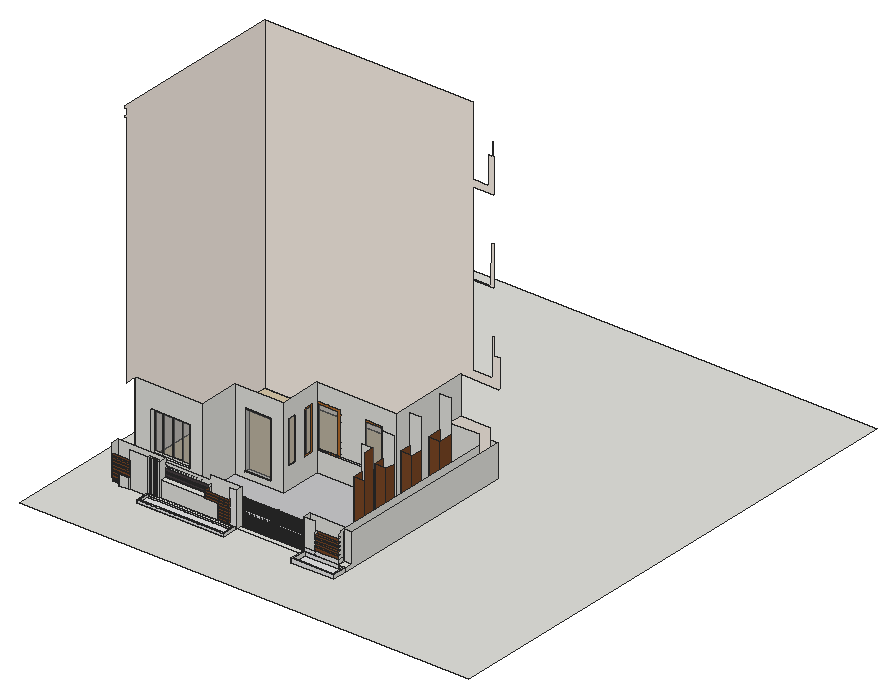
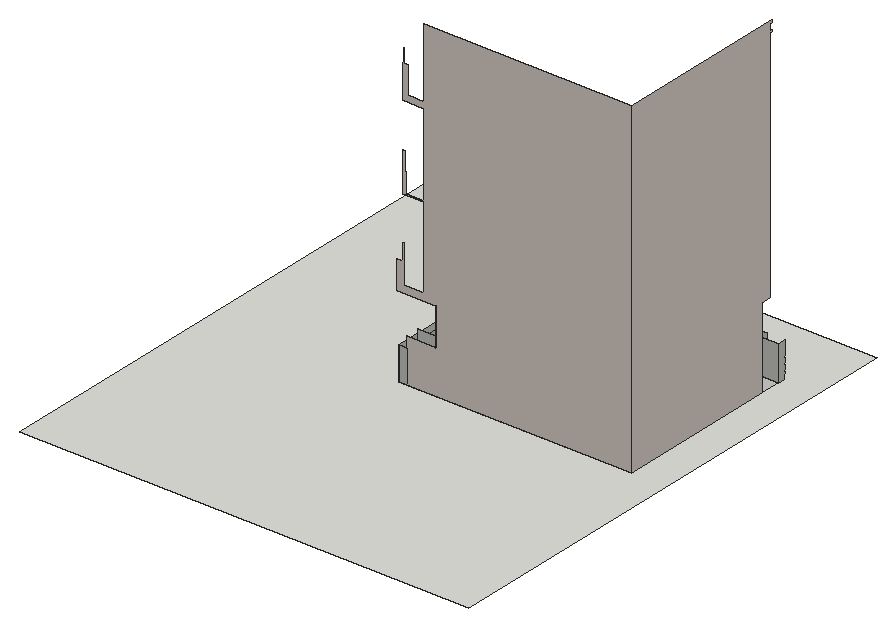
# SketchUp Ruby script. Lengths in inches.
U = 1.inch
M = Sketchup.active_model
def pt(a) = Geom::Point3d.new(a.map { |v| v * U })
def face(e, loops, mat)
  f = e.add_face(loops[0].map { |a| pt(a) })
  loops[1..].each { |l| e.add_face(l.map { |a| pt(a) }).erase! }
  f.material = f.back_material = mat if mat
  f
end
# faces: each face lists its corners as indices into pts; further lists are holes
def faces(e, pts, list, mat = nil) = list.each { |f| face(e, (f[0].is_a?(Array) ? f : [f]).map { |l| l.map { |i| pts[i] } }, mat) }
# xy, xz, yz: faces in a plane at the given z, y or x. An outline is a flat list of corners, or four numbers for a rectangle; further outlines are holes
def ring(l) = l.size == 4 ? [[l[0], l[1]], [l[2], l[1]], [l[2], l[3]], [l[0], l[3]]] : l.each_slice(2).to_a
def flat(e, list, mat, &to3) = list.each { |f| face(e, (f[0].is_a?(Array) ? f : [f]).map { |l| ring(l).map { |u, v| to3.(u, v) } }, mat) }
def xy(e, z, list, mat = nil) = flat(e, list, mat) { |x, y| [x, y, z] }
def xz(e, y, list, mat = nil) = flat(e, list, mat) { |x, z| [x, y, z] }
def yz(e, x, list, mat = nil) = flat(e, list, mat) { |y, z| [x, y, z] }
def lines(e, pts, list) = list.each { |a, b| e.add_line(pt(pts[a]), pt(pts[b])) }
# prism: a flat outline (further loops are holes) pulled along v
def prism(e, loops, v, mat = nil)
  f = face(e, loops, mat); d = Geom::Vector3d.new(v.map { |x| x * U })
  f.pushpull(f.normal.samedirection?(d) ? d.length : -d.length)
end
def box(e, o, s, mat = nil) = prism(e, [[o, [o[0] + s[0], o[1], o[2]], [o[0] + s[0], o[1] + s[1], o[2]], [o[0], o[1] + s[1], o[2]]]], [0, 0, s[2]], mat)
def at(x, y, z, deg = 0) = Geom::Transformation.translation(pt([x, y, z])) * Geom::Transformation.rotation(ORIGIN, Z_AXIS, deg.degrees)
def axes(o, x, y, z) = Geom::Transformation.new([*x, 0, *y, 0, *z, 0, *pt(o).to_a, 1])
def part(name) = M.definitions.add(name)
# library, detail: a bought-in or finely detailed component or shape, given as its bounding box
def library(name, o, s) = part(name).tap { |d| box(d.entities, o, s) }
def detail(e, o, s) = box(e.add_group.entities, o, s)
def put(e, d, t, mat = nil) = e.add_instance(d, t).tap { |i| i.material = mat if mat }
def group(e, t, mat = nil) = e.add_group.tap { |g| g.transformation = t; g.material = mat if mat }.entities
root = M.entities
M.materials.add("Color_008").color = [30, 30, 30]
M.materials.add("[0009_Linen]").color = [250, 240, 230]
M.materials.add("[0055_LightGoldenrodYellow]").color = [250, 250, 210]
M.materials.add("[0134_DimGray]").color = [105, 105, 105]
M.materials.add("[Asphalt New]").color = [67, 60, 62]
M.materials.add("[Field Square Tile]").color = [217, 201, 169]
M.materials.add("[Polished Concrete New]").color = [200, 200, 203]
M.materials.add("[Polished Concrete Old]").color = [229, 229, 229]
M.materials.add("[Translucent Glass Gray]").color = [128, 128, 128]
M.materials["[Translucent Glass Gray]"].alpha = 0.5
M.materials.add("[Wood Bamboo]").color = [177, 105, 43]
M.materials.add("[Wood Veneer 01]").color = [120, 70, 37]
c1 = part("Gate slat")
box(c1.entities,[0,0,-2.03],[1.97,0.97,40.94])
c2 = part("Gate frame member")
box(c2.entities,[0,0,0],[1.9,0.97,93.54])
c3 = part("Gate bar")
box(c3.entities,[2.95,0,-2.03],[0.99,0.97,40.94])
c4 = part("Slatted gate panel")
p = [[42.85,0.97,43.31],[42.85,0.97,44.29]]
lines(c4.entities,p,[[0,1]])
put(c4.entities,c1,axes([3.9375,0,86.61],[0,0,-1],[0,1,0],[1,0,0]),"Color_008")
put(c4.entities,c2,axes([87.6,0,0],[1,0,0],[0,1,0],[0,0,0.92593]),"Color_008")
put(c4.entities,c1,axes([48.6875,0,86.61],[0,0,-1],[0,1,0],[1,0,0]),"Color_008")
put(c4.entities,c2,axes([0,0,0],[1,0,0],[0,1,0],[0,0,0.92593]),"Color_008")
put(c4.entities,c2,axes([42.85,0,0],[1,0,0],[0,1,0],[0,0,0.92593]),"Color_008")
put(c4.entities,c2,axes([44.75,0,0],[1,0,0],[0,1,0],[0,0,0.92593]),"Color_008")
put(c4.entities,c3,axes([3.9375,0,87.11],[0,0,-1],[0,1,0],[1,0,0]),"[0134_DimGray]")
put(c4.entities,c3,axes([48.6875,0,87.11],[0,0,-1],[0,1,0],[1,0,0]),"[0134_DimGray]")
put(c4.entities,c1,axes([48.6875,0,82.68],[0,0,-1],[0,1,0],[1,0,0]),"Color_008")
put(c4.entities,c3,axes([48.6875,0,83.17],[0,0,-1],[0,1,0],[1,0,0]),"[0134_DimGray]")
put(c4.entities,c3,axes([3.9375,0,83.17],[0,0,-1],[0,1,0],[1,0,0]),"[0134_DimGray]")
put(c4.entities,c1,axes([3.9375,0,82.68],[0,0,-1],[0,1,0],[1,0,0]),"Color_008")
put(c4.entities,c3,axes([48.6875,0,75.3],[0,0,-1],[0,1,0],[1,0,0]),"[0134_DimGray]")
put(c4.entities,c1,axes([48.6875,0,78.74],[0,0,-1],[0,1,0],[1,0,0]),"Color_008")
put(c4.entities,c1,axes([48.6875,0,74.8],[0,0,-1],[0,1,0],[1,0,0]),"Color_008")
put(c4.entities,c3,axes([48.6875,0,79.23],[0,0,-1],[0,1,0],[1,0,0]),"[0134_DimGray]")
put(c4.entities,c3,axes([3.9375,0,75.3],[0,0,-1],[0,1,0],[1,0,0]),"[0134_DimGray]")
put(c4.entities,c1,axes([3.9375,0,78.74],[0,0,-1],[0,1,0],[1,0,0]),"Color_008")
put(c4.entities,c3,axes([3.9375,0,79.23],[0,0,-1],[0,1,0],[1,0,0]),"[0134_DimGray]")
put(c4.entities,c1,axes([3.9375,0,74.8],[0,0,-1],[0,1,0],[1,0,0]),"Color_008")
put(c4.entities,c3,axes([48.6875,0,67.42],[0,0,-1],[0,1,0],[1,0,0]),"[0134_DimGray]")
put(c4.entities,c3,axes([3.9375,0,63.48],[0,0,-1],[0,1,0],[1,0,0]),"[0134_DimGray]")
put(c4.entities,c3,axes([48.6875,0,71.36],[0,0,-1],[0,1,0],[1,0,0]),"[0134_DimGray]")
put(c4.entities,c3,axes([3.9375,0,67.42],[0,0,-1],[0,1,0],[1,0,0]),"[0134_DimGray]")
put(c4.entities,c1,axes([3.9375,0,70.87],[0,0,-1],[0,1,0],[1,0,0]),"Color_008")
put(c4.entities,c1,axes([48.6875,0,70.87],[0,0,-1],[0,1,0],[1,0,0]),"Color_008")
put(c4.entities,c1,axes([48.6875,0,66.93],[0,0,-1],[0,1,0],[1,0,0]),"Color_008")
put(c4.entities,c1,axes([48.6875,0,59.06],[0,0,-1],[0,1,0],[1,0,0]),"Color_008")
put(c4.entities,c1,axes([3.9375,0,55.12],[0,0,-1],[0,1,0],[1,0,0]),"Color_008")
put(c4.entities,c1,axes([3.9375,0,62.99],[0,0,-1],[0,1,0],[1,0,0]),"Color_008")
put(c4.entities,c3,axes([3.9375,0,59.55],[0,0,-1],[0,1,0],[1,0,0]),"[0134_DimGray]")
put(c4.entities,c1,axes([3.9375,0,66.93],[0,0,-1],[0,1,0],[1,0,0]),"Color_008")
put(c4.entities,c1,axes([48.6875,0,62.99],[0,0,-1],[0,1,0],[1,0,0]),"Color_008")
put(c4.entities,c3,axes([48.6875,0,59.55],[0,0,-1],[0,1,0],[1,0,0]),"[0134_DimGray]")
put(c4.entities,c3,axes([48.6875,0,63.48],[0,0,-1],[0,1,0],[1,0,0]),"[0134_DimGray]")
put(c4.entities,c1,axes([3.9375,0,59.06],[0,0,-1],[0,1,0],[1,0,0]),"Color_008")
put(c4.entities,c3,axes([3.9375,0,71.36],[0,0,-1],[0,1,0],[1,0,0]),"[0134_DimGray]")
put(c4.entities,c3,axes([3.9375,0,33.96],[0,0,-1],[0,1,0],[1,0,0]),"[0134_DimGray]")
put(c4.entities,c3,axes([48.6875,0,33.96],[0,0,-1],[0,1,0],[1,0,0]),"[0134_DimGray]")
put(c4.entities,c1,axes([3.9375,0,29.53],[0,0,-1],[0,1,0],[1,0,0]),"Color_008")
put(c4.entities,c3,axes([3.9375,0,26.08],[0,0,-1],[0,1,0],[1,0,0]),"[0134_DimGray]")
put(c4.entities,c1,axes([3.9375,0,33.46],[0,0,-1],[0,1,0],[1,0,0]),"Color_008")
put(c4.entities,c1,axes([48.6875,0,29.53],[0,0,-1],[0,1,0],[1,0,0]),"Color_008")
put(c4.entities,c3,axes([48.6875,0,30.02],[0,0,-1],[0,1,0],[1,0,0]),"[0134_DimGray]")
put(c4.entities,c1,axes([3.9375,0,25.59],[0,0,-1],[0,1,0],[1,0,0]),"Color_008")
put(c4.entities,c1,axes([48.6875,0,25.59],[0,0,-1],[0,1,0],[1,0,0]),"Color_008")
put(c4.entities,c1,axes([48.6875,0,33.46],[0,0,-1],[0,1,0],[1,0,0]),"Color_008")
put(c4.entities,c1,axes([3.9375,0,49.7],[0,0,-1],[0,1,0],[1,0,0]),"Color_008")
put(c4.entities,c3,axes([48.6875,0,26.08],[0,0,-1],[0,1,0],[1,0,0]),"[0134_DimGray]")
put(c4.entities,c3,axes([3.9375,0,30.02],[0,0,-1],[0,1,0],[1,0,0]),"[0134_DimGray]")
put(c4.entities,c1,axes([3.9375,0,5.91],[0,0,-1],[0,1,0],[1,0,0]),"Color_008")
put(c4.entities,c1,axes([48.6875,0,13.78],[0,0,-1],[0,1,0],[1,0,0]),"Color_008")
put(c4.entities,c3,axes([48.6875,0,10.33],[0,0,-1],[0,1,0],[1,0,0]),"[0134_DimGray]")
put(c4.entities,c3,axes([3.9375,0,6.4],[0,0,-1],[0,1,0],[1,0,0]),"[0134_DimGray]")
put(c4.entities,c1,axes([3.9375,0,13.78],[0,0,-1],[0,1,0],[1,0,0]),"Color_008")
put(c4.entities,c1,axes([48.6875,0,21.65],[0,0,-1],[0,1,0],[1,0,0]),"Color_008")
put(c4.entities,c1,axes([48.6875,0,5.91],[0,0,-1],[0,1,0],[1,0,0]),"Color_008")
put(c4.entities,c3,axes([48.6875,0,22.15],[0,0,-1],[0,1,0],[1,0,0]),"[0134_DimGray]")
put(c4.entities,c1,axes([48.6875,0,1.97],[0,0,-1],[0,1,0],[1,0,0]),"Color_008")
put(c4.entities,c1,axes([48.6875,0,9.84],[0,0,-1],[0,1,0],[1,0,0]),"Color_008")
put(c4.entities,c3,axes([48.6875,0,6.4],[0,0,-1],[0,1,0],[1,0,0]),"[0134_DimGray]")
put(c4.entities,c1,axes([3.9375,0,9.84],[0,0,-1],[0,1,0],[1,0,0]),"Color_008")
put(c4.entities,c3,axes([3.9375,0,10.33],[0,0,-1],[0,1,0],[1,0,0]),"[0134_DimGray]")
put(c4.entities,c3,axes([3.9375,0,22.15],[0,0,-1],[0,1,0],[1,0,0]),"[0134_DimGray]")
put(c4.entities,c1,axes([3.9375,0,1.97],[0,0,-1],[0,1,0],[1,0,0]),"Color_008")
put(c4.entities,c3,axes([3.9375,0,18.21],[0,0,-1],[0,1,0],[1,0,0]),"[0134_DimGray]")
put(c4.entities,c3,axes([3.9375,0,14.27],[0,0,-1],[0,1,0],[1,0,0]),"[0134_DimGray]")
put(c4.entities,c1,axes([3.9375,0,21.65],[0,0,-1],[0,1,0],[1,0,0]),"Color_008")
put(c4.entities,c3,axes([48.6875,0,18.21],[0,0,-1],[0,1,0],[1,0,0]),"[0134_DimGray]")
put(c4.entities,c1,axes([3.9375,0,17.72],[0,0,-1],[0,1,0],[1,0,0]),"Color_008")
put(c4.entities,c1,axes([48.6875,0,17.72],[0,0,-1],[0,1,0],[1,0,0]),"Color_008")
put(c4.entities,c3,axes([48.6875,0,14.27],[0,0,-1],[0,1,0],[1,0,0]),"[0134_DimGray]")
put(c4.entities,c1,axes([3.9375,0,44.29],[0,0,-1],[0,1,0],[1,0,0]),"Color_008")
put(c4.entities,c1,axes([3.9375,0,38.88],[0,0,-1],[0,1,0],[1,0,0]),"Color_008")
put(c4.entities,c1,axes([48.6875,0,49.7],[0,0,-1],[0,1,0],[1,0,0]),"Color_008")
put(c4.entities,c1,axes([48.6875,0,44.29],[0,0,-1],[0,1,0],[1,0,0]),"Color_008")
put(c4.entities,c1,axes([48.6875,0,38.88],[0,0,-1],[0,1,0],[1,0,0]),"Color_008")
put(c4.entities,c1,axes([48.6875,0,55.12],[0,0,-1],[0,1,0],[1,0,0]),"Color_008")
c5 = part("Porton+casa (1)")
put(c5.entities,c4,axes([-601.47,309.65,-100.84],[0.96774,0,0],[0,1,0],[0,0,1]),"[0055_LightGoldenrodYellow]")
xy(root,0,[[[0,0,1600.8125,1814.75],[253.79,202.52,253.79,250.88,189.05,250.88,189.05,246.44,153.49,246.44,153.49,258.13,124.44,258.13,124.44,934.03,954.26,934.03,954.26,258.13,948.8,258.13,948.8,208.47,808.9,208.47,808.9,258.13,565.2,258.13,565.2,202.52]],[[253.79,202.52,565.2,250.88],[259.75,208.48,559.24,244.93]],[153.49,246.44,189.05,246.44,189.05,250.88,153.49,258.13],[189.05,250.88,189.05,258.13,153.49,258.13],[189.05,250.88,253.79,258.13],
  [253.79,250.88,262.32,258.13],[262.32,250.88,268.72,258.13],[268.72,250.88,274.39,258.13],[274.39,250.88,281.75,258.13],[281.75,250.88,287.33,258.13],
  [287.33,250.88,295.6,258.13],[295.6,250.88,565.2,258.13],[124.44,258.13,565.2,279.68],[565.2,258.13,803.4375,284.25],[803.4375,258.13,927.67,284.25]])
xy(root,0,[[927.67,258.13,954.26,258.13,954.26,934.03,124.44,934.03,124.44,354.61,366.22,354.61,366.22,498.96,538.78,498.96,538.78,649.35,821.9,649.35,821.9,884.53,927.67,884.53]],"[Field Square Tile]")
xy(root,0,[[[124.44,279.68,565.2,279.68,565.2,284.25,927.67,284.25,927.67,884.53,821.9,884.53,821.9,649.35,538.78,649.35,538.78,498.96,366.22,498.96,366.22,354.61,124.44,354.61],[850.45,757.51,889.83,807.18],[850.45,631.85,889.83,672.61],[850.45,424,889.83,460.43],[850.45,516.77,889.83,551.84]]],"[Polished Concrete New]")
xy(root,0,[[808.9,208.47,948.8,258.13],[259.75,208.48,559.24,244.93]],"[Polished Concrete Old]")
xy(root,9,[[[253.79,202.52,565.2,250.88],[259.75,208.48,559.24,244.93]]])
xy(root,11,[[499.46,254.69,541.39,258.13]],"[Wood Veneer 01]")
xy(root,14.0625,[[803.4375,203.57,954.26,203.57,954.26,258.13,948.8,258.13,948.8,208.47,808.9,208.47,808.9,258.13,803.4375,258.13],[927.67,258.13,954.26,284.25]])
xy(root,16.59,[[124.44,250.88,153.49,258.13]],"[Wood Veneer 01]")
xy(root,17.34,[[499.46,254.69,541.39,258.13]],"[Wood Veneer 01]")
xy(root,22,[[499.46,254.69,541.39,258.13]],"[Wood Veneer 01]")
xy(root,23.56,[[124.44,250.88,153.49,258.13]],"[Wood Veneer 01]")
xy(root,25.04,[[406.18,498.96,495.01,511.34]])
xy(root,27.96,[[124.44,250.88,153.49,258.13]],"[Wood Veneer 01]")
xy(root,28.34,[[499.46,254.69,541.39,258.13]],"[Wood Veneer 01]")
xy(root,30.9375,[[499.46,254.69,541.39,258.13]],"[Wood Veneer 01]")
xy(root,34.93,[[124.44,250.88,153.49,258.13]],"[Wood Veneer 01]")
xy(root,35.5625,[[153.49,246.44,189.05,246.44,189.05,250.88,153.49,258.13],[189.05,250.88,189.05,258.13,153.49,258.13]])
xy(root,37.28,[[499.46,254.69,541.39,258.13]],"[Wood Veneer 01]")
xy(root,39.34,[[124.44,250.88,189.05,258.13]],"[Wood Veneer 01]")
xy(root,40.05,[[842.13,258.13,927.67,268.51]],"[Wood Veneer 01]")
xy(root,40.75,[[499.46,254.69,541.39,258.13]],"[Wood Veneer 01]")
xy(root,46.08,[[842.13,258.13,927.67,268.51]],"[Wood Veneer 01]")
xy(root,46.31,[[124.44,250.88,189.05,258.13]],"[Wood Veneer 01]")
xy(root,47.09,[[499.46,254.69,541.39,258.13]],"[Wood Veneer 01]")
xy(root,50.71,[[124.44,250.88,189.05,258.13]],"[Wood Veneer 01]")
xy(root,51.0625,[[499.46,254.69,541.39,258.13]],"[Wood Veneer 01]")
xy(root,52.08,[[842.13,258.13,927.67,268.51]],"[Wood Veneer 01]")
xy(root,57.4,[[499.46,254.69,541.39,258.13]],"[Wood Veneer 01]")
xy(root,57.68,[[124.44,250.88,189.05,258.13]],"[Wood Veneer 01]")
xy(root,60.12,[[842.13,258.13,927.67,268.51]],"[Wood Veneer 01]")
xy(root,62,[[295.6,258.13,455.17,279.68]])
xy(root,62,[[455.17,254.69,499.46,258.13],[499.46,254.69,541.39,258.13]],"[Wood Veneer 01]")
xy(root,62.09,[[124.44,250.88,189.05,258.13]],"[Wood Veneer 01]")
xy(root,63.22,[[181.21,354.61,321.33,367.17]])
xy(root,65.71,[[842.13,258.13,927.67,268.51]],"[Wood Veneer 01]")
xy(root,68.34,[[455.17,254.69,541.39,258.13]],"[Wood Veneer 01]")
xy(root,69.06,[[124.44,250.88,189.05,258.13]],"[Wood Veneer 01]")
xy(root,69.63,[[295.6,273.26,454.72,279.68]],"[Asphalt New]")
xy(root,71.52,[[455.17,254.69,541.39,258.13]],"[Wood Veneer 01]")
xy(root,73.46,[[124.44,250.88,189.05,258.13]],"[Wood Veneer 01]")
xy(root,73.74,[[842.13,258.13,927.67,268.51]],"[Wood Veneer 01]")
xy(root,77.18,[[295.6,273.26,454.72,279.68]],"[Asphalt New]")
xy(root,77.86,[[455.17,254.69,541.39,258.13]],"[Wood Veneer 01]")
xy(root,79.64,[[842.13,258.13,927.67,268.51]],"[Wood Veneer 01]")
xy(root,80.43,[[124.44,250.88,189.05,258.13]],"[Wood Veneer 01]")
xy(root,81.05,[[455.17,254.69,541.39,258.13]],"[Wood Veneer 01]")
xy(root,84.84,[[124.44,250.88,189.05,258.13]],"[Wood Veneer 01]")
xy(root,85.63,[[295.6,273.26,455.17,279.68]],"[Asphalt New]")
xz(root,202.52,[[253.79,0,565.2,9]],"[Polished Concrete Old]")
xz(root,203.57,[[803.4375,0,954.26,14.0625]],"[Polished Concrete Old]")
xz(root,208.47,[[808.9,0,948.8,14.0625]])
xz(root,208.48,[[259.75,0,559.24,9]])
xz(root,244.93,[[259.75,0,262.32,9],[262.32,0,268.72,9],[268.72,0,274.39,9],[274.39,0,281.75,9],[281.75,0,287.33,9],
  [287.33,0,295.6,9]])
xz(root,244.93,[[295.6,0,559.24,9]],"[Polished Concrete Old]")
xz(root,246.44,[[153.49,0,189.05,35.5625]])
xz(root,250.88,[[189.05,0,253.79,124],[253.79,0,262.32,9],[262.32,0,268.72,9],[268.72,0,274.39,9],[274.39,0,281.75,9],
  [281.75,0,287.33,9],[287.33,0,295.6,9],[295.6,0,565.2,9],[262.32,9,268.72,124],[274.39,9,281.75,124],
  [287.33,9,295.6,124]])
xz(root,250.88,[[124.44,16.59,153.49,23.56],[124.44,27.96,153.49,34.93],[124.44,39.34,189.05,46.31],[124.44,50.71,189.05,57.68],[124.44,62.09,189.05,69.06],
  [124.44,73.46,189.05,80.43],[124.44,84.84,189.05,91.81]],"[Wood Veneer 01]")
xz(root,254.69,[[499.46,11,541.39,17.34],[499.46,22,541.39,28.34],[499.46,30.9375,541.39,37.28],[499.46,40.75,541.39,47.09],[499.46,51.0625,541.39,57.4],
  [455.17,62,541.39,68.34],[455.17,71.52,541.39,77.86],[455.17,81.05,541.39,87.39]],"[Wood Veneer 01]")
xz(root,258.13,[[124.44,0,153.49,0.81],[253.79,0,262.32,124],[268.72,0,274.39,124],[281.75,0,287.33,124],[295.6,0,499.46,62],
  [803.4375,0,808.9,14.0625],[948.8,0,954.26,14.0625],[803.4375,28.01,842.13,124]])
xz(root,258.13,[[541.39,0,565.2,124],[808.9,0,927.67,14.0625],[927.67,0,948.8,14.0625],[803.4375,14.0625,842.13,28.01],[842.13,14.0625,927.67,28.01]],"[Polished Concrete Old]")
xz(root,258.13,[[499.46,0,541.39,11],[124.44,0.81,153.49,5.21],[124.44,5.21,153.49,12.18],[124.44,12.18,153.49,16.59],[499.46,17.34,541.39,22],
  [124.44,23.56,153.49,27.96],[842.13,28.01,927.67,40.05],[499.46,28.34,541.39,30.9375],[124.44,34.93,153.49,34.93,153.49,35.5625,189.05,35.5625,189.05,39.34,124.44,39.34],[499.46,37.28,541.39,40.75],
  [842.13,46.08,927.67,52.08],[124.44,46.31,189.05,50.71],[499.46,47.09,541.39,51.0625],[499.46,57.4,541.39,62],[124.44,57.68,189.05,62.09],
  [842.13,60.12,927.67,65.71],[455.17,68.34,541.39,71.52],[124.44,69.06,189.05,73.46],[842.13,73.74,927.67,79.64],[455.17,77.86,541.39,81.05],
  [124.44,80.43,189.05,84.84]],"[Wood Veneer 01]")
xz(root,268.51,[[842.13,40.05,927.67,46.08],[842.13,52.08,927.67,60.12],[842.13,65.71,927.67,73.74],[842.13,79.64,927.67,87.68]],"[Wood Veneer 01]")
xz(root,273.26,[[295.6,69.63,454.72,77.18],[295.6,85.63,455.17,94.84]],"[Asphalt New]")
xz(root,279.68,[[[124.44,0,124.44,124,295.6,124,295.6,109.42,455.17,109.42,455.17,124,565.2,124,565.2,0],[295.6,62,455.17,62,455.17,85.63,295.6,85.63,295.6,77.18,454.72,77.18,454.72,69.63,295.6,69.63],[295.6,94.84,455.17,100.52]]])
xz(root,284.25,[[803.4375,0,927.67,124],[927.67,14.0625,954.26,116.625]])
xz(root,354.61,[[[124.44,0,366.22,287.75],[181.21,63.22,321.33,209.22]]])
xz(root,367.17,[[[181.21,63.22,321.33,203.35],[187.8,69.82,314.73,196.75]],[214.99,69.82,216.62,196.75],[251.27,69.82,253.38,196.75],[284.06,69.82,286.73,196.75]])
xz(root,367.17,[[187.8,69.82,214.99,196.75],[216.62,69.82,251.27,196.75],[253.38,69.82,284.06,196.75],[286.73,69.82,314.73,196.75]],"[Translucent Glass Gray]")
xz(root,424,[[850.45,0,889.83,195.12]],"[Wood Veneer 01]")
xz(root,460.43,[[850.45,0,889.83,284.1875]])
xz(root,498.96,[[[366.22,0,538.78,287.75],[402.41,21.26,498.78,225.95]],[[402.41,21.26,498.78,225.95],[406.18,25.04,495.01,222.18]]])
xz(root,498.96,[[406.18,25.04,495.01,222.18]],"[Translucent Glass Gray]")
xz(root,516.77,[[850.45,0,889.83,195.12]],"[Wood Veneer 01]")
xz(root,551.84,[[850.45,0,889.83,284.375]])
xz(root,631.85,[[850.45,0,889.83,185.07]],"[Wood Veneer 01]")
xz(root,649.35,[[538.78,0,821.9,0,821.9,287.75,538.78,287.75,538.78,229.23,622.09,229.23,622.09,78.92,707.38,78.92,707.38,229.23,773.82,229.23,773.82,73.42,538.78,73.42],[622.09,73.42,707.38,78.92]])
xz(root,649.35,[[546.55,78.92,614.33,220.68],[712.89,78.92,768.3125,223.73]],"[Translucent Glass Gray]")
xz(root,649.35,[[538.78,73.42,622.09,73.42,622.09,78.92,614.33,78.92,614.33,73.7,546.55,73.7,546.55,78.92,538.78,78.92],[[707.38,73.42,773.82,229.23],[712.89,78.92,768.3125,223.73]],[546.55,73.7,614.33,78.92],[538.78,78.92,546.55,78.92,546.55,220.68,614.33,220.68,614.33,78.92,622.09,78.92,622.09,229.23,538.78,229.23]],"[Wood Bamboo]")
xz(root,672.61,[[850.45,0,889.83,290.83]])
xz(root,757.51,[[850.45,0,889.83,174.63]],"[Wood Veneer 01]")
xz(root,807.18,[[850.45,0,889.83,290.83]])
xz(root,884.53,[[821.9,0,927.67,155.125]])
xz(root,934.03,[[927.67,0,954.26,116.625]])
xz(root,934.03,[[124.44,0,124.44,1173.6875,865.53,1173.6875,865.53,926.8125,924.26,926.8125,924.26,1023.625,936.15,1023.625,936.15,1071.875,936.87,1071.875,936.87,1023.625,941.71,1023.625,941.71,903.4375,865.61,903.4375,865.61,609.59,930.23,609.59,930.23,679.4,933.62,679.4,933.62,745.21,941.71,745.21,941.71,605.77,865.61,605.77,865.61,316.375,937.99,316.375,937.99,449.0625,941.71,449.0625,941.71,390.25,962.51,390.25,962.51,386.71,960.69,386.71,960.69,385,962.51,385,962.51,381.83,960.69,381.83,960.69,379.32,962.51,379.32,962.51,376.14,960.69,376.14,960.69,373.63,962.51,373.63,962.51,370.46,960.69,370.46,960.69,367.94,962.51,367.94,962.51,364.77,960.69,364.77,960.69,362.25,962.51,362.25,962.51,359.08,960.69,359.08,960.69,356.57,962.51,356.57,962.51,353.39,960.69,353.39,960.69,350.88,962.51,350.88,962.51,347.71,960.69,347.71,960.69,345.19,962.51,345.19,962.51,342.02,960.69,342.02,960.69,339.5,962.51,339.5,962.51,336.33,960.69,336.33,960.69,333.82,962.51,333.82,962.51,330.64,960.69,330.64,960.69,328.13,962.51,328.13,962.51,324.96,960.69,324.96,960.69,322.44,962.51,322.44,962.51,319.27,960.69,319.27,960.69,316.75,962.51,316.75,962.51,313.58,960.69,313.58,960.69,311.07,962.51,311.07,962.51,307.89,960.69,307.89,960.69,305.38,962.51,305.38,962.51,302.21,960.69,302.21,960.69,299.69,962.51,299.69,962.51,296.52,960.69,296.52,960.69,294,962.51,294,962.51,290.83,960.69,290.83,960.69,287.75,821.9,287.75,821.9,155.125,927.67,155.125,927.67,0]],"[0009_Linen]")
yz(root,124.44,[[258.13,0,258.13,16.59,250.88,16.59,250.88,23.56,258.13,23.56,258.13,27.96,250.88,27.96,250.88,34.93,258.13,34.93,258.13,39.34,250.88,39.34,250.88,46.31,258.13,46.31,258.13,50.71,250.88,50.71,250.88,57.68,258.13,57.68,258.13,62.09,250.88,62.09,250.88,69.06,258.13,69.06,258.13,73.46,250.88,73.46,250.88,80.43,258.13,80.43,258.13,84.84,250.88,84.84,250.88,91.81,258.13,91.81,258.13,96.21,250.88,96.21,250.88,103.18,258.13,103.18,258.13,107.59,250.88,107.59,250.88,114.56,258.13,114.56,258.13,117.42,250.88,117.42,250.88,124,279.68,124,279.68,0]])
yz(root,124.44,[[354.61,0,354.61,287.75,316.98,287.75,316.98,1137.19,311.67,1137.19,311.67,1142.63,316.98,1142.63,316.98,1165.85,311.67,1165.85,311.67,1173.6875,934.03,1173.6875,934.03,0]],"[0009_Linen]")
yz(root,153.49,[[246.44,0,258.13,16.59],[246.44,16.59,250.88,23.56],[250.88,16.59,258.13,23.56],[246.44,23.56,258.13,27.96],[246.44,27.96,250.88,34.93],
  [250.88,27.96,258.13,34.93],[246.44,34.93,258.13,35.5625]])
yz(root,181.21,[[354.61,63.22,367.17,203.35]])
yz(root,189.05,[[246.44,0,250.88,35.5625],[250.88,35.5625,258.13,39.34],[250.88,46.31,258.13,50.71],[250.88,57.68,258.13,62.09],[250.88,69.06,258.13,73.46],
  [250.88,80.43,258.13,84.84]])
yz(root,253.79,[[202.52,0,250.88,9],[250.88,0,258.13,124]])
yz(root,259.75,[[208.48,0,244.93,9]])
yz(root,262.32,[[250.88,0,258.13,124]])
yz(root,268.72,[[250.88,0,258.13,124]])
yz(root,274.39,[[250.88,0,258.13,124]])
yz(root,281.75,[[250.88,0,258.13,124]])
yz(root,287.33,[[250.88,0,258.13,124]])
yz(root,295.6,[[250.88,0,258.13,0,258.13,62,279.68,62,279.68,69.63,273.26,69.63,273.26,77.18,279.68,77.18,279.68,85.63,273.26,85.63,273.26,94.84,279.68,94.84,279.68,100.52,273.26,100.52,273.26,109.42,279.68,109.42,279.68,124,250.88,124]])
yz(root,321.33,[[354.61,63.22,367.17,203.35]])
yz(root,366.22,[[354.61,0,498.96,287.75]])
yz(root,406.18,[[498.96,25.04,511.34,222.18]])
yz(root,454.72,[[273.26,69.63,279.68,77.18]])
yz(root,455.17,[[273.26,62,279.68,85.63],[258.13,68.34,273.26,71.52],[258.13,77.86,273.26,81.05],[273.26,85.63,279.68,94.84]])
yz(root,455.17,[[254.69,62,273.26,68.34],[254.69,71.52,273.26,77.86],[254.69,81.05,273.26,87.39]],"[Wood Veneer 01]")
yz(root,495.01,[[498.96,25.04,511.34,222.18]])
yz(root,499.46,[[254.69,11,258.13,17.34],[254.69,22,258.13,28.34],[254.69,30.9375,258.13,37.28],[254.69,40.75,258.13,47.09],[254.69,51.0625,258.13,57.4]],"[Wood Veneer 01]")
yz(root,538.78,[[[498.96,0,649.35,287.75],[592.87,73.78,627.31,228.65],[521.04,73.78,553.46,228.65]]])
yz(root,538.78,[[523.66,76.4,550.84,226.03],[598.17,79.08,622.01,223.36]],"[Translucent Glass Gray]")
yz(root,538.78,[[[521.04,73.78,553.46,228.65],[523.66,76.4,550.84,226.03]],[[592.87,73.78,627.31,228.65],[598.17,79.08,622.01,223.36]]],"[Wood Bamboo]")
yz(root,541.39,[[254.69,11,258.13,17.34],[254.69,22,258.13,28.34],[254.69,30.9375,258.13,37.28],[254.69,40.75,258.13,47.09],[254.69,51.0625,258.13,57.4],
  [254.69,62,258.13,68.34],[254.69,71.52,258.13,77.86],[254.69,81.05,258.13,87.39]],"[Wood Veneer 01]")
yz(root,559.24,[[208.48,0,244.93,9]])
yz(root,565.2,[[202.52,0,250.88,9],[258.13,0,279.68,124]])
yz(root,803.4375,[[203.57,0,258.13,14.0625],[258.13,0,284.25,124]])
yz(root,808.9,[[208.47,0,258.13,14.0625]])
yz(root,821.9,[[649.35,0,884.53,0,884.53,155.125,934.03,155.125,934.03,287.75,649.35,287.75]])
yz(root,842.13,[[258.13,40.05,268.51,46.08],[258.13,52.08,268.51,60.12],[258.13,65.71,268.51,73.74],[258.13,79.64,268.51,87.68]])
yz(root,850.45,[[424,0,460.43,195.12],[516.77,0,551.84,195.12],[631.85,0,672.61,185.07],[757.51,0,807.18,174.63]],"[Wood Veneer 01]")
yz(root,889.83,[[424,0,460.43,284.1875],[516.77,0,551.84,0,551.84,191.02,516.77,195.12],[631.85,0,672.61,0,672.61,180.31,631.85,185.07],[757.51,0,807.18,174.63]],"[Wood Veneer 01]")
yz(root,927.67,[[258.13,0,284.25,14.0625],[284.25,0,884.53,116.625],[258.13,14.0625,284.25,28.01],[258.13,28.01,284.25,28.01,284.25,116.625,268.51,116.625,268.51,109.73,258.13,109.73,258.13,101.99,268.51,101.99,268.51,93.96,258.13,93.96,258.13,87.68,268.51,87.68,268.51,79.64,258.13,79.64,258.13,73.74,268.51,73.74,268.51,65.71,258.13,65.71,258.13,60.12,268.51,60.12,268.51,52.08,258.13,52.08,258.13,46.08,268.51,46.08,268.51,40.05,258.13,40.05]])
yz(root,948.8,[[208.47,0,258.13,14.0625]])
yz(root,954.26,[[203.57,0,258.13,14.0625],[258.13,0,934.03,0,934.03,116.625,284.25,116.625,284.25,14.0625,258.13,14.0625]])
p = [[153.49,258.13,0],[189.05,250.88,0],[189.05,250.88,35.5625],[153.49,258.13,35.5625],[153.49,258.13,34.93],[153.49,258.13,27.96],
  [153.49,258.13,23.56],[153.49,258.13,16.59],[153.49,258.13,12.18],[153.49,258.13,5.21],[153.49,258.13,0.81],[189.05,258.13,27.96],
  [189.05,258.13,34.93],[189.05,258.13,16.59],[189.05,258.13,23.56],[189.05,258.13,5.21],[189.05,258.13,12.18],[189.05,258.13,0.81]]
faces(root,p,[[0,1,2,3,4,5,6,7,8,9,10]])
lines(root,p,[[11,5],[4,12],[13,7],[6,14],[15,9],[8,16],[10,17]])
put(root,c5,axes([2219.24,-29.96,110.09],[2.75,0,0],[0,1,0],[0,0,1.0918]))
